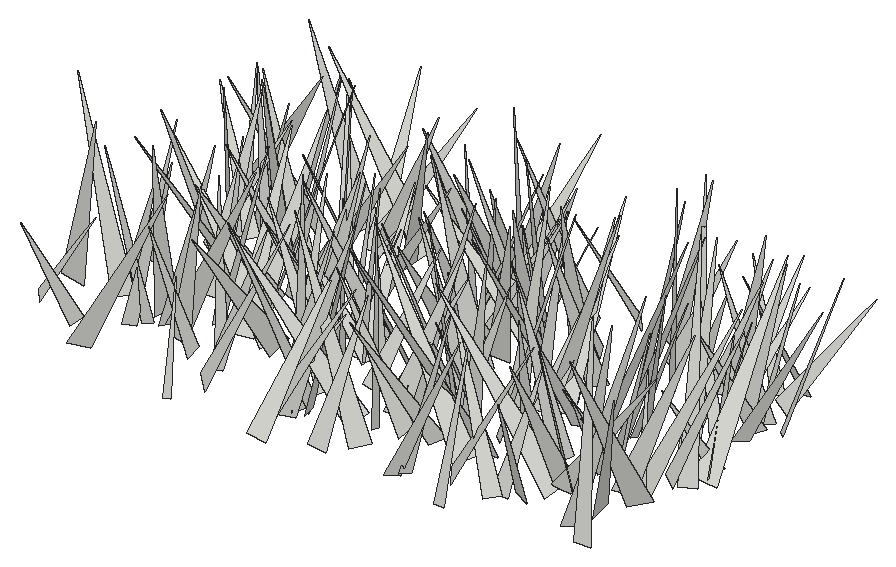
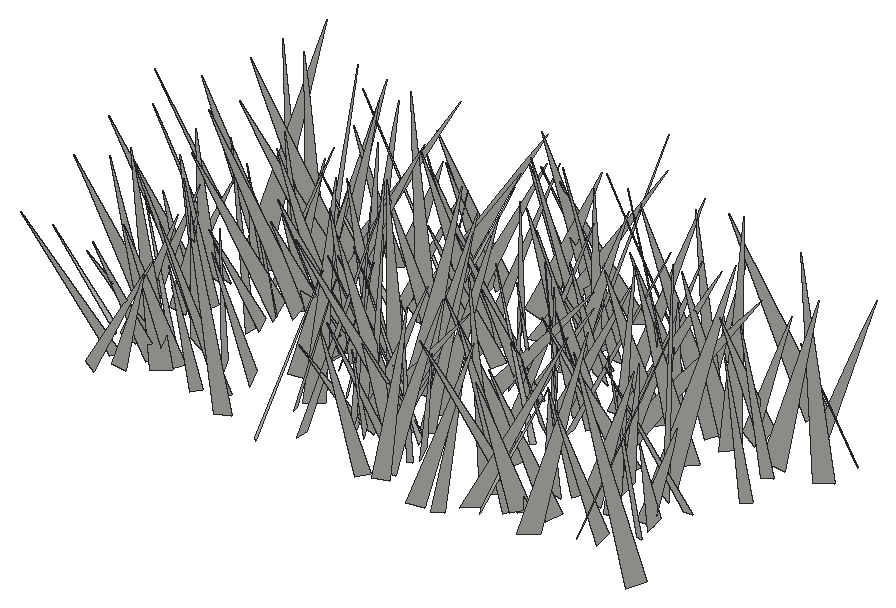
# SketchUp Ruby script. Lengths in inches.
U = 1.inch
M = Sketchup.active_model
def pt(a) = Geom::Point3d.new(a.map { |v| v * U })
def face(e, loops, mat)
  f = e.add_face(loops[0].map { |a| pt(a) })
  loops[1..].each { |l| e.add_face(l.map { |a| pt(a) }).erase! }
  f.material = f.back_material = mat if mat
  f
end
# faces: each face lists its corners as indices into pts; further lists are holes
def faces(e, pts, list, mat = nil) = list.each { |f| face(e, (f[0].is_a?(Array) ? f : [f]).map { |l| l.map { |i| pts[i] } }, mat) }
# xy, xz, yz: faces in a plane at the given z, y or x. An outline is a flat list of corners, or four numbers for a rectangle; further outlines are holes
def ring(l) = l.size == 4 ? [[l[0], l[1]], [l[2], l[1]], [l[2], l[3]], [l[0], l[3]]] : l.each_slice(2).to_a
def flat(e, list, mat, &to3) = list.each { |f| face(e, (f[0].is_a?(Array) ? f : [f]).map { |l| ring(l).map { |u, v| to3.(u, v) } }, mat) }
def xy(e, z, list, mat = nil) = flat(e, list, mat) { |x, y| [x, y, z] }
def xz(e, y, list, mat = nil) = flat(e, list, mat) { |x, z| [x, y, z] }
def yz(e, x, list, mat = nil) = flat(e, list, mat) { |y, z| [x, y, z] }
def lines(e, pts, list) = list.each { |a, b| e.add_line(pt(pts[a]), pt(pts[b])) }
# prism: a flat outline (further loops are holes) pulled along v
def prism(e, loops, v, mat = nil)
  f = face(e, loops, mat); d = Geom::Vector3d.new(v.map { |x| x * U })
  f.pushpull(f.normal.samedirection?(d) ? d.length : -d.length)
end
def box(e, o, s, mat = nil) = prism(e, [[o, [o[0] + s[0], o[1], o[2]], [o[0] + s[0], o[1] + s[1], o[2]], [o[0], o[1] + s[1], o[2]]]], [0, 0, s[2]], mat)
def at(x, y, z, deg = 0) = Geom::Transformation.translation(pt([x, y, z])) * Geom::Transformation.rotation(ORIGIN, Z_AXIS, deg.degrees)
def axes(o, x, y, z) = Geom::Transformation.new([*x, 0, *y, 0, *z, 0, *pt(o).to_a, 1])
def part(name) = M.definitions.add(name)
# library, detail: a bought-in or finely detailed component or shape, given as its bounding box
def library(name, o, s) = part(name).tap { |d| box(d.entities, o, s) }
def detail(e, o, s) = box(e.add_group.entities, o, s)
def put(e, d, t, mat = nil) = e.add_instance(d, t).tap { |i| i.material = mat if mat }
def group(e, t, mat = nil) = e.add_group.tap { |g| g.transformation = t; g.material = mat if mat }.entities
root = M.entities
c1 = part("fur_instance\#9")
p = [[0.8125,0,1.79],[0.67,-0.02,1.48],[0,-0.11,0],[0,0.11,0]]
faces(c1.entities,p,[[0,1,2,3]])
put(root,c1,axes([514.55,259.96,-21.66],[0.6459,3.9486,0.07217],[3.68247,-0.62859,1.43463],[-1.42692,0.16515,3.73504]))
put(root,c1,axes([540.52,264.04,-21.66],[-1.15105,-5.30671,0.17],[-5.09537,1.15297,1.49093],[1.49242,-0.15644,5.22142]))
put(root,c1,axes([532.19,261.12,-21.66],[5.41003,-2.25588,0.78895],[-2.38957,-5.13634,1.69936],[-0.03699,1.87321,5.60977]))
put(root,c1,axes([522.25,259.52,-21.66],[-1.13308,6.40977,0.66119],[6.08836,1.28481,-2.02171],[2.11049,-0.26515,6.18722]))
put(root,c1,axes([526.18,260.875,-21.66],[-0.72846,5.64896,1.65026],[5.62241,1.15927,-1.48642],[1.73859,-1.38206,5.49837]))
put(root,c1,axes([503.7,264.25,-21.66],[3.91388,-2.85851,1.41513],[-2.09693,-3.9939,-2.26798],[-2.40345,-1.17037,4.2832]))
put(root,c1,axes([537.02,259.88,-21.66],[1.91748,5.33638,0.31642],[5.10909,-1.9283,1.55969],[-1.57297,0.24194,5.4517]))
put(root,c1,axes([505.78,261.86,-21.66],[5.9864,-4.39629,0.74457],[-4.35138,-5.48795,2.58196],[0.97326,2.50473,6.96403]))
put(root,c1,axes([522.33,265.16,-21.66],[-7.22673,-3.69522,1.05519],[-3.3656,7.17065,2.06111],[1.85494,-1.38592,7.85061]))
put(root,c1,axes([521.2,262.11,-21.66],[4.19059,5.13354,0.34706],[4.85008,-3.79176,-2.47669],[1.71767,-1.81771,6.14657]))
put(root,c1,axes([525.96,265.35,-21.66],[-7.44265,2.94787,0.75024],[2.95668,6.54484,3.6151],[-0.71474,-3.62229,7.14241]))
put(root,c1,axes([535.19,263.45,-21.66],[5.77692,4.11347,0.10405],[3.90568,-5.42514,-2.37018],[1.29504,-1.98782,6.68399]))
put(root,c1,axes([545.58,265.83,-21.66],[6.93671,-0.62868,0.23505],[-0.51232,-6.5363,-2.3628],[-0.4336,-2.33453,6.55213]))
put(root,c1,axes([547.41,261.68,-21.66],[1.24745,7.40868,1.63783],[7.39275,-1.56046,1.42803],[-1.70827,-1.34297,7.376]))
put(root,c1,axes([515.06,263.05,-21.66],[5.08074,5.57509,0.64514],[5.46993,-4.72427,-2.25231],[1.25607,-1.97773,7.19879]))
put(root,c1,axes([532.65,261.9,-21.66],[5.29795,0.17393,1.896],[-0.4687,-5.31448,1.7972],[-1.84537,1.84915,4.98684]))
put(root,c1,axes([531.67,266.46,-21.66],[2.44843,-5.51273,0.60157],[-4.8536,-2.44839,-2.68234],[-2.6823,-0.60174,5.40279]))
put(root,c1,axes([521.76,262.91,-21.66],[6.06814,-4.77445,2.10475],[-5.2154,-5.64781,2.22478],[-0.15808,3.05854,7.39379]))
put(root,c1,axes([541.93,266.96,-21.66],[4.15216,-5.25606,0.30062],[-4.95254,-4.0295,-2.04756],[-1.78575,-1.04593,6.37763]))
put(root,c1,axes([528.15,262.85,-21.66],[-2.68904,7.46116,1.26428],[7.06219,1.99214,3.26422],[-2.71897,-2.20471,7.22805]))
put(root,c1,axes([539.2,263.43,-21.66],[-0.86303,4.80618,1.97762],[4.83833,1.47497,-1.47315],[1.8976,-1.57489,4.65553]))
put(root,c1,axes([512.11,265.7,-21.66],[-5.24413,-0.63684,1.6828],[-0.10679,5.28634,1.66778],[1.7961,-1.54509,5.01248]))
put(root,c1,axes([546.99,268.14,-21.66],[4.52461,-6.7861,0.00105],[-6.53347,-4.35651,-2.20405],[-1.83437,-1.22185,7.85273]))
put(root,c1,axes([539.01,262.92,-21.66],[-2.13966,5.92839,0.3544],[5.56639,1.87053,2.31645],[-2.07043,-1.09766,5.86157]))
put(root,c1,axes([542.28,266.91,-21.66],[-3.66849,-5.82093,1.22872],[-5.44278,3.86666,2.06783],[2.40191,-0.1285,6.56241]))
put(root,c1,axes([541.65,266.14,-21.66],[-7.78216,2.50032,0.23977],[2.4235,7.26917,2.85602],[-0.66011,-2.78901,7.65877]))
put(root,c1,axes([529.37,266.14,-21.66],[-6.5147,0.26004,1.16019],[0.55336,6.38259,1.67669],[1.05235,-1.74639,6.3006]))
put(root,c1,axes([520.51,264.24,-21.66],[2.74298,6.25055,1.8619],[6.47418,-2.36552,-1.59662],[0.78801,-2.32269,6.63657]))
put(root,c1,axes([516,269.7,-21.66],[6.60243,-3.6292,1.16999],[-2.40466,-5.77841,-4.35427],[-2.95933,-3.40161,6.14845]))
put(root,c1,axes([510.49,266.42,-21.66],[0.32033,-6.88611,1.90206],[-6.92731,0.16595,1.76741],[1.74605,1.92169,6.66313]))
put(root,c1,axes([499.67,265.39,-21.66],[3.27011,3.05252,0.13659],[2.8317,-2.95233,-1.81533],[1.14804,-1.41282,4.08853]))
put(root,c1,axes([534.22,267.75,-21.66],[-2.23996,-8.03771,0.28468],[-7.44594,1.96073,-3.22749],[-3.04036,1.11981,7.69451]))
put(root,c1,axes([514.61,264.79,-21.66],[4.76351,-2.22786,1.63166],[-2.67424,-4.53288,1.61806],[-0.68857,2.19233,5.00362]))
put(root,c1,axes([545.27,263.12,-21.66],[7.73551,0.03019,2.73159],[-1.01366,-7.58581,2.95441],[-2.53672,3.12332,7.14916]))
put(root,c1,axes([522.16,264.07,-21.66],[-7.61718,0.0241,1.98426],[-0.51537,7.57673,-2.07045],[1.91631,2.1335,7.33043]))
put(root,c1,axes([519.91,265.63,-21.66],[0.48143,3.7055,0.846],[3.27794,0.02687,-1.98307],[1.92393,-0.97302,3.16701]))
put(root,c1,axes([522.75,264.32,-21.66],[7.20277,3.49638,1.97973],[3.12762,-7.42996,1.74287],[-2.5223,0.77133,7.81454]))
put(root,c1,axes([535.77,267.12,-21.66],[-2.3451,-4.39084,0.71964],[-4.31416,2.04482,-1.58228],[-1.08875,1.35503,4.71968]))
put(root,c1,axes([534.6,265.64,-21.66],[-4.02573,7.19257,0.41274],[6.48293,3.4104,3.80141],[-3.14246,-2.17854,7.31361]))
put(root,c1,axes([541.81,266.46,-21.66],[4.55,-4.60588,0.41001],[-4.16176,-3.82822,3.1795],[2.01545,2.49305,5.6398]))
put(root,c1,axes([533.07,267.97,-21.66],[0.67729,-7.55263,2.0847],[-7.70125,-0.25666,1.57216],[1.44182,2.17688,7.41817]))
put(root,c1,axes([507.36,268.89,-21.66],[7.0973,-2.99001,1.53723],[-2.6894,-7.20395,-1.59536],[-2.01752,-0.91535,7.53436]))
put(root,c1,axes([521.97,267.27,-21.66],[-5.92654,3.46188,1.28835],[3.68281,5.72588,1.55549],[0.28525,-1.99951,6.68498]))
put(root,c1,axes([500.04,268.42,-21.66],[1.15039,-7.47242,1.55869],[-7.41634,-0.72104,2.01691],[1.80677,1.79806,7.28646]))
put(root,c1,axes([527.53,265.23,-21.66],[-6.50203,-1.48304,1.94789],[-2.15091,6.10063,-2.53495],[1.1693,2.97539,6.16846]))
put(root,c1,axes([509.24,267.82,-21.66],[5.85705,-5.48153,0.51052],[-5.36351,-5.5136,2.33363],[1.24121,2.04104,7.67505]))
put(root,c1,axes([507.39,266.93,-21.66],[-2.16703,-5.16397,2.37315],[-5.48971,1.24499,-2.30381],[-1.47021,2.96275,5.10441]))
put(root,c1,axes([542.55,270.04,-21.66],[3.43107,-2.8474,0.0502],[-2.64084,-3.2106,-1.6126],[-1.06592,-1.21113,4.15686]))
put(root,c1,axes([543.73,270.6,-21.66],[-4.54437,-2.07997,0.71062],[-1.49312,4.11891,2.50752],[1.61302,-2.04715,4.32318]))
put(root,c1,axes([539.58,269.47,-21.66],[-6.14349,2.42883,3.06477],[3.31416,6.26335,1.67969],[2.07568,-2.81172,6.38908]))
put(root,c1,axes([511.83,268.57,-21.66],[6.05057,5.41917,1.99571],[5.77348,-5.74186,-1.9125],[-0.1309,-2.76104,7.89425]))
put(root,c1,axes([536.23,270.26,-21.66],[5.5268,-1.95543,1.04999],[-1.67194,-5.52102,-1.48142],[-1.45972,-1.07995,5.67227]))
put(root,c1,axes([527.36,267.42,-21.66],[-2.26569,5.88907,2.62757],[5.5866,3.18358,-2.31806],[3.22106,-1.37923,5.86866]))
put(root,c1,axes([513.45,266.93,-21.66],[-5.70107,0.73605,0.76728],[0.48907,5.53142,-1.67238],[0.94409,1.57933,5.49974]))
put(root,c1,axes([508.53,267.57,-21.66],[6.30569,-0.68619,2.05979],[-1.17683,-6.39727,1.4715],[-1.82446,1.75482,6.16987]))
put(root,c1,axes([531.38,269.62,-21.66],[-5.94217,-4.1756,0.21971],[-4.13273,5.80684,-1.41225],[-0.63601,1.27993,7.12394]))
put(root,c1,axes([545.28,268.57,-21.66],[4.70932,-5.02611,1.74089],[-5.27526,-4.11549,2.38842],[0.68127,2.87596,6.46026]))
put(root,c1,axes([506.62,266.04,-21.66],[-6.46453,1.71895,1.7422],[0.79023,6.12289,-3.109],[2.31637,2.70842,5.92275]))
put(root,c1,axes([532.46,267.73,-21.66],[-6.42625,-2.81034,1.42452],[-3.14557,5.90814,-2.53441],[0.18076,2.90169,6.53999]))
put(root,c1,axes([503.95,268.75,-21.66],[-2.60972,7.0339,1.93347],[7.14895,2.0575,2.16424],[-1.45142,-2.51309,7.18348]))
put(root,c1,axes([515.29,269.82,-21.66],[-6.72983,3.60579,0.05795],[3.45053,6.40273,2.3226],[-1.04828,-2.07339,7.27309]))
put(root,c1,axes([503.29,270.16,-21.66],[0.14432,-5.01914,1.5992],[-4.96199,0.40759,1.72702],[1.76858,1.55311,4.71487]))
put(root,c1,axes([519.85,266.64,-21.66],[1.21236,6.8418,0.01969],[6.58716,-1.17263,1.87473],[-1.84929,0.30844,6.6907]))
put(root,c1,axes([527.87,268.22,-21.66],[7.54644,-1.30772,2.23251],[-1.88035,-7.50036,1.96263],[-1.77721,2.38276,7.40318]))
put(root,c1,axes([531.01,269.57,-21.66],[4.31663,-3.25233,1.38409],[-3.53279,-4.03972,1.52536],[-0.11299,2.05661,5.185]))
put(root,c1,axes([525.99,269.45,-21.66],[3.23121,-4.00646,1.7311],[-4.24322,-2.37965,2.41277],[1.02152,2.78831,4.54653]))
put(root,c1,axes([513.48,272.05,-21.66],[-2.19661,-7.3796,0.4517],[-6.30745,1.62463,-4.13089],[-3.85727,1.54587,6.49764]))
put(root,c1,axes([546.67,268.61,-21.66],[0.48963,4.22721,0.04806],[3.94805,-0.47454,1.51627],[-1.51146,0.12987,3.97618]))
put(root,c1,axes([512.29,274.11,-21.66],[6.08199,-2.63161,2.26399],[-1.13407,-5.82276,-3.72169],[-3.281,-2.8656,5.48316]))
put(root,c1,axes([524,269.15,-21.66],[-0.28996,5.60424,1.15409],[5.32871,0.68543,-1.98963],[2.08431,-0.97272,5.24719]))
put(root,c1,axes([540.14,271.59,-21.66],[-0.32261,-5.78503,1.74562],[-5.69921,0.87225,1.8374],[2.00818,1.5461,5.49497]))
put(root,c1,axes([546.14,269.48,-21.66],[3.48936,7.09192,0.65775],[6.9322,-3.21357,-2.12629],[1.63479,-1.51038,7.61247]))
put(root,c1,axes([518.51,273.14,-21.66],[0.56796,-5.36738,0.34113],[-5.01782,-0.65229,-1.90884],[-1.93561,0.11605,5.04853]))
put(root,c1,axes([521.62,271.9,-21.66],[-4.01783,2.35497,0.3103],[2.27352,3.63609,1.84258],[-0.68795,-1.73727,4.27712]))
put(root,c1,axes([537.57,273.72,-21.66],[-1.57704,-7.74459,0.50786],[-7.45096,1.36569,-2.31124],[-2.17253,0.93802,7.55804]))
put(root,c1,axes([516.91,273.6,-21.66],[-7.35388,-1.92649,0.06127],[-1.88282,7.23164,1.39751],[0.41243,-1.33667,7.47248]))
put(root,c1,axes([513.2,269.4,-21.66],[-3.83392,6.10516,1.11787],[5.9137,3.99214,-1.52073],[1.88436,-0.10697,7.04694]))
put(root,c1,axes([520.8125,274.48,-21.66],[-7.04471,-1.4589,1.32068],[-0.96261,6.83613,2.41686],[1.71638,-2.15394,6.77607]))
put(root,c1,axes([520.48,270.61,-21.66],[-5.01766,-1.40088,1.70753],[-1.93126,4.83928,-1.7049],[1.07162,2.16194,4.92267]))
put(root,c1,axes([511.08,269.67,-21.66],[-5.97598,0.81352,1.54005],[0.17172,5.75229,-2.37225],[1.73323,2.235,5.54496]))
put(root,c1,axes([517.9375,270.6875,-21.66],[7.25129,-2.23194,2.73946],[-2.93898,-7.28136,1.84704],[-1.96177,2.6585,7.35875]))
put(root,c1,axes([515.91,271.94,-21.66],[3.27115,-5.93629,2.22387],[-6.24966,-2.60094,2.25],[1.06155,2.98013,6.39355]))
put(root,c1,axes([528.81,272.96,-21.66],[1.01091,-5.94061,2.30759],[-6.04054,-1.63799,-1.57056],[-2.03168,1.91413,5.81775]))
put(root,c1,axes([507.83,275.125,-21.66],[3.07442,-7.15508,0.96712],[-6.88437,-3.22185,-1.95131],[-2.1762,0.08396,7.5392]))
put(root,c1,axes([546.61,271.68,-21.66],[3.72746,5.46093,0.78491],[5.42353,-3.45332,-1.72965],[1.01153,-1.60767,6.38153]))
put(root,c1,axes([534.61,269.0625,-21.66],[5.37795,5.75,0.47067],[5.40496,-5.24661,2.33794],[-2.01755,1.27162,7.51791]))
put(root,c1,axes([548.32,274.57,-21.66],[2.70067,-3.13661,0.88183],[-2.51329,-2.73437,-2.02883],[-2.07348,-0.77102,3.60774]))
put(root,c1,axes([523.68,270.85,-21.66],[-4.92435,-0.05312,0.24709],[-0.15186,4.47527,-2.06445],[0.20202,2.06935,4.47102]))
put(root,c1,axes([502.33,273.51,-21.66],[0.76926,-4.66703,1.07076],[-4.59745,-0.41678,1.48633],[1.33832,1.25083,4.49041]))
put(root,c1,axes([541.43,273.21,-21.66],[3.4231,3.63538,1.50249],[3.93251,-3.11512,-1.42212],[0.09387,-2.06666,4.78656]))
put(root,c1,axes([525.06,276.84,-21.66],[5.40671,-4.03304,0.21931],[-3.53675,-4.90438,-2.9974],[-1.95061,-2.2864,6.04264]))
put(root,c1,axes([521.23,271.6,-21.66],[2.56304,5.03632,1.18387],[4.82189,-2.80423,1.49027],[-1.87495,-0.32715,5.45094]))
put(root,c1,axes([508.32,272.16,-21.66],[-2.56408,6.91655,2.55207],[6.94878,3.17004,-1.60986],[2.46298,-1.74312,7.19872]))
put(root,c1,axes([524.03,273.08,-21.66],[-5.38862,-5.55187,0.24968],[-4.68183,4.34761,-4.37054],[-2.99434,3.19341,6.38427]))
put(root,c1,axes([540.44,271.85,-21.66],[8.13769,0.92636,1.08085],[0.65484,-8.00564,1.93114],[-1.26395,1.81658,7.95932]))
put(root,c1,axes([517.89,276.0625,-21.66],[5.66121,2.03663,0.41958],[1.99596,-4.98096,-2.75306],[0.58316,-2.72311,5.34956]))
put(root,c1,axes([521.08,271.87,-21.66],[-3.49002,4.97532,0.38419],[4.70613,3.43753,-1.76559],[1.65943,0.71499,5.81522]))
put(root,c1,axes([527.9,275.61,-21.66],[2.50523,-6.92108,2.84903],[-7.08461,-3.16179,-1.45116],[-2.41383,2.09672,7.21607]))
put(root,c1,axes([548.07,271.72,-21.66],[0.30584,8.28043,0.48557],[7.987,-0.4251,2.21855],[-2.2381,-0.38549,7.98355]))
put(root,c1,axes([541.33,275.86,-21.66],[6.22131,1.299,1.34326],[1.60809,-6.10017,-1.54868],[-0.95174,-1.81575,6.1639]))
put(root,c1,axes([506.64,276.43,-21.66],[-4.19902,-6.23031,2.61813],[-6.01537,4.8505,1.89504],[3.08005,0.97931,7.27031]))
put(root,c1,axes([532.84,273.1,-21.66],[-6.71814,2.72987,2.53139],[2.23652,7.13443,-1.75826],[2.97626,0.8008,7.03521]))
put(root,c1,axes([527.91,277.38,-21.66],[2.36593,-6.95857,0.28973],[-6.83072,-2.25873,1.53056],[1.359,0.76137,7.18865]))
put(root,c1,axes([548.5625,273.63,-21.66],[-4.5247,0.14497,1.56827],[-0.47946,4.4174,-1.79167],[1.5002,1.84904,4.15738]))
put(root,c1,axes([534.73,274.53,-21.66],[7.47756,-1.51643,1.55812],[-1.8154,-7.42558,1.48539],[-1.19651,1.78955,7.48379]))
put(root,c1,axes([534.61,273.63,-21.66],[-3.66435,5.27166,1.90181],[4.6134,4.12758,-2.55233],[3.18179,0.08644,5.89097]))
put(root,c1,axes([541.47,272.73,-21.66],[7.3603,1.92647,1.4977],[1.22652,-7.03518,3.02165],[-2.10951,2.63124,6.98247]))
put(root,c1,axes([533.68,274.38,-21.66],[-6.0255,1.4926,2.28597],[0.94971,6.33899,-1.63567],[2.5596,1.16168,5.98825]))
put(root,c1,axes([524.07,279.2,-21.66],[6.25747,-1.85529,1.59771],[-1.00282,-5.94215,-2.97253],[-2.23363,-2.52972,5.81052]))
put(root,c1,axes([516.98,274.49,-21.66],[5.31118,5.11176,2.74997],[4.78098,-5.96627,1.85658],[-3.29161,-0.41778,7.13385]))
put(root,c1,axes([548.43,273.04,-21.66],[-1.16046,8.00046,0.20395],[7.87345,1.17823,-1.41992],[1.43448,0.00519,7.95851]))
put(root,c1,axes([535.15,278.57,-21.66],[2.99002,-5.93259,1.12286],[-5.76165,-3.17812,-1.449],[-1.8055,0.31717,6.48354]))
put(root,c1,axes([531.17,278.61,-21.66],[-4.0085,-3.44331,0.94309],[-3.06456,4.04605,1.74695],[1.83147,-0.76613,4.98725]))
put(root,c1,axes([534.1,275.56,-21.66],[-5.43034,-1.89464,0.64767],[-1.9986,5.01546,-2.08529],[-0.12137,2.18018,5.36002]))
put(root,c1,axes([541.21,274.79,-21.66],[4.47299,1.54799,0.88013],[1.09405,-4.26651,1.94385],[-1.40498,1.60599,4.31572]))
put(root,c1,axes([518.46,274.24,-21.66],[1.86893,4.92203,0.04113],[4.36091,-1.67616,2.42774],[-2.28266,0.8277,4.67176]))
put(root,c1,axes([528.74,279.9,-21.66],[6.44625,-4.17663,0.34492],[-3.99481,-6.31514,-1.81045],[-1.26676,-1.33867,7.46462]))
put(root,c1,axes([527.57,278.01,-21.66],[-0.38653,-3.78857,0.47263],[-3.40937,0.1287,-1.7566],[-1.71837,0.59684,3.37891]))
put(root,c1,axes([545.21,275.38,-21.66],[-6.19625,3.45387,1.64148],[3.0912,6.3638,-1.72156],[2.25127,0.76815,6.88178]))
put(root,c1,axes([535.02,275.68,-21.66],[5.43487,-1.88004,3.06705],[-2.9758,-5.47185,1.91904],[-2.02138,3.00059,5.42123]))
put(root,c1,axes([512.02,274.07,-21.66],[6.2923,4.31715,0.79405],[3.75537,-6.01297,2.93303],[-2.27277,2.01685,7.04472]))
put(root,c1,axes([507.96,280.32,-21.66],[-1.88375,-7.99896,1.23534],[-7.80751,2.13018,1.88761],[2.13359,0.73274,7.99805]))
put(root,c1,axes([546.625,276.74,-21.66],[-1.63602,4.97918,0.62205],[4.87533,1.42244,1.43652],[-1.18757,-1.0199,5.04036]))
put(root,c1,axes([547.03,280.26,-21.66],[2.87484,-4.36178,0.57915],[-3.91954,-2.85297,-2.03053],[-1.99945,-0.67874,4.81319]))
put(root,c1,axes([512.45,275.22,-21.66],[3.92721,6.27569,0.86047],[6.07775,-4.01843,1.56873],[-1.78486,0.12492,7.23508]))
put(root,c1,axes([535.59,274.375,-21.66],[-4.59589,5.78444,0.11594],[5.4804,4.40003,-2.28044],[1.8543,1.33244,7.02721]))
put(root,c1,axes([510.55,275.0625,-21.66],[-4.56425,4.1816,0.8559],[3.58274,4.43445,-2.55936],[2.31998,1.37862,5.63629]))
put(root,c1,axes([504.38,276.95,-21.66],[2.28513,5.39499,0.34939],[5.12885,-2.04337,-1.99232],[1.70965,-1.08097,5.50984]))
put(root,c1,axes([532.2,280.67,-21.66],[6.58115,-3.41587,1.26301],[-3.10443,-6.62563,-1.74311],[-1.90417,-1.00387,7.20703]))
put(root,c1,axes([516.94,278.48,-21.66],[4.74645,-3.63152,0.20608],[-3.44873,-4.38539,2.15263],[1.15614,1.82746,5.57521]))
put(root,c1,axes([509.33,276.97,-21.66],[-6.71,0.21588,0.88951],[-0.0468,6.49159,-1.92847],[0.91413,1.91692,6.43053]))
put(root,c1,axes([543.35,278.3,-21.66],[2.52048,5.79703,1.2985],[5.75928,-2.03853,-2.07834],[1.45681,-1.97061,5.96983]))
put(root,c1,axes([525.625,278.48,-21.66],[4.10268,4.53992,0.30052],[4.35228,-3.79801,-2.04106],[1.3262,-1.58032,5.76861]))
put(root,c1,axes([511.33,279.69,-21.66],[1.52564,-3.34819,0.07276],[-3.07421,-1.36842,1.48995],[1.32851,0.67846,3.36423]))
put(root,c1,axes([546.86,278.69,-21.66],[5.8068,-2.41673,0.19711],[-2.36119,-5.5195,1.88633],[0.55156,1.81463,6.0001]))
put(root,c1,axes([528.11,280.47,-21.66],[-5.02457,3.67244,0.21301],[3.24783,4.25941,3.17608],[-1.72736,-2.67378,5.35216]))
put(root,c1,axes([525.98,279.1,-21.66],[3.52755,5.08967,0.59914],[4.90233,-3.13928,-2.19532],[1.49362,-1.71683,5.79042]))
put(root,c1,axes([543.72,280.74,-21.66],[4.89387,1.35478,0.49174],[1.44124,-4.60961,-1.64362],[-0.00784,-1.71558,4.80457]))
put(root,c1,axes([528.08,281.85,-21.66],[-6.05203,-3.65216,2.90127],[-3.20675,6.70926,1.75646],[3.38709,-0.1736,6.84691]))
put(root,c1,axes([532.67,282.09,-21.66],[-3.8372,-2.33717,0.79383],[-2.01321,3.81242,1.493],[1.42812,-0.90538,4.23762]))
put(root,c1,axes([523.78,280.33,-21.66],[5.98281,3.47845,0.55141],[3.51313,-5.81778,-1.41742],[0.2481,-1.50052,6.77381]))
put(root,c1,axes([510.14,279.76,-21.66],[-1.88222,6.06948,1.49765],[6.0067,1.32242,2.18977],[-1.73238,-2.00921,5.96542]))
put(root,c1,axes([504.8,281.49,-21.66],[3.94876,4.2171,2.00571],[4.64379,-3.26946,-2.26834],[0.4919,-2.98768,5.31331]))
put(root,c1,axes([508.03,283.68,-21.66],[-6.16351,-3.9605,0.27898],[-3.73191,5.95492,2.08903],[1.35509,-1.6142,7.02213]))
put(root,c1,axes([505.7,279.73,-21.66],[-2.49681,4.68547,0.3153],[4.52882,2.308,1.56527],[-1.24213,-1.0033,5.07323]))
put(root,c1,axes([527.52,281.21,-21.66],[-0.80032,5.57612,2.90873],[5.9333,-0.30294,2.21326],[-2.08561,-3.00158,5.18026]))
put(root,c1,axes([545.11,281.22,-21.66],[0.56131,-6.10589,2.64479],[-6.41112,0.21442,1.85565],[1.78167,2.69518,5.8441]))
put(root,c1,axes([527.89,280.16,-21.66],[3.6249,6.4726,3.15784],[6.5149,-4.45394,1.65071],[-3.06961,-1.8095,7.23254]))
put(root,c1,axes([515.9,283.15,-21.66],[7.05622,-1.23215,0.51957],[-1.10047,-6.93599,-1.50315],[-0.75967,-1.39725,7.0035]))
put(root,c1,axes([546.875,281.53,-21.66],[-1.11932,5.12608,2.18052],[5.30702,0.30525,2.00664],[-1.6932,-2.43194,4.84799]))
put(root,c1,axes([525.21,280.9,-21.66],[6.77248,-2.83159,1.61361],[-3.13932,-6.6674,1.47599],[-0.87537,2.00399,7.19067]))
put(root,c1,axes([522.54,282.91,-21.66],[-1.98967,-4.65459,1.69235],[-4.24096,2.54317,2.00863],[2.55803,0.59592,4.64644]))
put(root,c1,axes([530.27,284.41,-21.66],[-7.65526,-2.65251,1.50577],[-2.23878,7.64939,2.09305],[2.07148,-1.53532,7.82675]))
put(root,c1,axes([524.98,279.68,-21.66],[0.81957,8.13408,0.73803],[7.68253,-0.51597,-2.84467],[2.77248,-0.97476,7.66439]))
put(root,c1,axes([505.1,279.58,-21.66],[-5.60466,1.1961,0.32776],[0.92969,5.05609,-2.5538],[0.82084,2.4404,5.13039]))
put(root,c1,axes([522.93,284.87,-21.66],[2.61621,-5.42084,0.25429],[-5.22177,-2.59146,-1.52055],[-1.47757,-0.43991,5.82391]))
put(root,c1,axes([524.6,282.89,-21.66],[-1.27388,-3.61865,0.59779],[-3.46584,0.98064,-1.44951],[-1.19998,1.0092,3.55195]))
put(root,c1,axes([542.63,283.4375,-21.66],[2.44609,-6.94499,1.47158],[-6.99231,-2.08787,1.76924],[1.22722,1.94671,7.14745]))
put(root,c1,axes([542.59,279.5625,-21.66],[1.27817,7.72916,0.81529],[7.27012,-1.48113,2.64386],[-2.74773,-0.32349,7.37453]))
put(root,c1,axes([539.55,280.73,-21.66],[-6.21182,-1.68937,2.27799],[-2.42044,6.01654,-2.13837],[1.47806,2.75267,6.07191]))
put(root,c1,axes([512.8125,280.42,-21.66],[-0.78819,5.89997,0.04998],[5.7265,0.75282,1.4401],[-1.42105,-0.23877,5.77555]))
put(root,c1,axes([510.75,282.79,-21.66],[4.20762,-3.32651,0.12048],[-3.15177,-3.91891,1.86887],[1.07075,1.53645,5.02763]))
put(root,c1,axes([537.28,280.64,-21.66],[5.41894,2.39891,1.8987],[1.67708,-5.5593,2.23748],[-2.55876,1.4367,5.48756]))
put(root,c1,axes([522.55,281.55,-21.66],[-5.22043,-0.84385,1.05571],[-1.17009,4.93002,-1.84535],[0.67639,2.01552,4.95577]))
put(root,c1,axes([528.24,281.05,-21.66],[3.83996,1.68055,0.1423],[1.49178,-3.54944,1.66307],[-0.78682,1.47206,3.84756]))
put(root,c1,axes([546.59,280.93,-21.66],[2.63197,4.07891,0.20518],[3.86496,-2.5665,1.44292],[-1.31973,0.61842,4.63495]))
put(root,c1,axes([527.16,281.7,-21.66],[3.31155,2.43431,1.59522],[1.82743,-3.61986,1.73033],[-2.2652,0.63849,3.72802]))
put(root,c1,axes([522.61,285.83,-21.66],[4.609,-3.3139,0.05026],[-3.15306,-4.41083,-1.68231],[-1.0211,-1.33793,5.42168]))
put(root,c1,axes([524.55,282.49,-21.66],[1.36791,4.73736,0.76135],[4.55305,-1.0318,-1.76027],[1.51392,-1.17738,4.60599]))
put(root,c1,axes([513.3125,283.76,-21.66],[4.4628,-4.8312,0.78242],[-4.8199,-4.15484,1.83716],[0.84924,1.80724,6.31521]))
put(root,c1,axes([542.03,282.58,-21.66],[3.72107,-3.56028,1.90501],[-4.03778,-3.30047,1.71878],[-0.03061,2.5656,4.85467]))
put(root,c1,axes([539.13,284.17,-21.66],[1.54528,-3.8993,0.59524],[-3.77652,-1.27799,1.43226],[1.13873,1.05307,3.94222]))
put(root,c1,axes([548.45,280.93,-21.66],[3.88995,3.95886,0.07672],[3.75671,-3.72392,1.68217],[-1.25122,1.12695,5.2891]))
put(root,c1,axes([537.33,283.51,-21.66],[1.43912,5.66343,2.07225],[5.60003,-0.46439,-2.61988],[2.23794,-2.47985,5.22319]))
put(root,c1,axes([544.11,281.53,-21.66],[-0.54715,4.89077,0.10405],[4.53126,0.54616,-1.84371],[1.84341,0.10915,4.56287]))
put(root,c1,axes([532.22,286.76,-21.66],[-4.33714,-4.09832,0.0827],[-3.81397,4.0787,2.10515],[1.50223,-1.4771,5.58349]))
put(root,c1,axes([515.79,285.1,-21.66],[-7.5943,2.08618,0.38061],[2.11361,7.33132,1.9887],[-0.17228,-2.01745,7.62041]))
put(root,c1,axes([501.11,286.39,-21.66],[2.01455,-7.63294,0.11302],[-6.59973,-1.68273,3.99311],[3.83642,1.11337,6.80994]))
put(root,c1,axes([510.69,285.49,-21.66],[-6.83352,3.26319,2.339],[3.80782,6.73136,1.73366],[1.27275,-2.61852,7.37155]))
put(root,c1,axes([535.85,285.58,-21.66],[-0.11111,-7.60969,2.49454],[-7.52897,0.94928,2.56048],[2.72852,2.30953,7.16685]))
put(root,c1,axes([506.48,283.1,-21.66],[5.33264,0.16428,1.51785],[-0.27785,-5.31816,1.55174],[-1.50122,1.56784,5.10452]))
put(root,c1,axes([546.19,283.69,-21.66],[1.31269,5.55847,0.82299],[4.82858,-0.68361,-3.08457],[2.8738,-1.39037,4.80678]))
put(root,c1,axes([517.03,286.91,-21.66],[4.74802,-2.11154,0.82126],[-1.70244,-4.58339,-1.94189],[-1.49491,-1.48682,4.81989]))
put(root,c1,axes([512.66,283.39,-21.66],[1.506,6.6666,0.93752],[6.04421,-0.91584,-3.19677],[2.9648,-1.51928,6.04088]))
put(root,c1,axes([543.68,282.86,-21.66],[-1.09311,5.26549,0.63584],[5.05113,1.23151,-1.51458],[1.61731,-0.28736,5.16007]))
put(root,c1,axes([515.3125,284.54,-21.66],[-5.46904,-3.01802,0.13387],[-2.92547,5.22183,-1.79189],[-0.75368,1.63119,5.98398]))
put(root,c1,axes([546.5,285.95,-21.66],[-1.81586,-4.37557,0.34615],[-4.20637,1.62778,-1.48984],[-1.25376,0.87607,4.49704]))
put(root,c1,axes([518.75,287.1,-21.66],[3.32641,-4.64571,1.36805],[-4.19977,-3.59363,-1.99171],[-2.41165,-0.14974,5.35544]))
put(root,c1,axes([544.98,284.86,-21.66],[-1.55107,4.41542,0.77186],[4.34501,1.28043,1.40671],[-1.10114,-1.16708,4.46351]))
put(root,c1,axes([523.87,286.1,-21.66],[2.085,-4.49657,0.98747],[-4.39792,-1.62495,1.88661],[1.36107,1.63764,4.58334]))
put(root,c1,axes([512.97,283.46,-21.66],[-3.56356,5.20391,0.71647],[5.00613,3.62664,-1.4419],[1.59144,0.24443,6.14008]))
